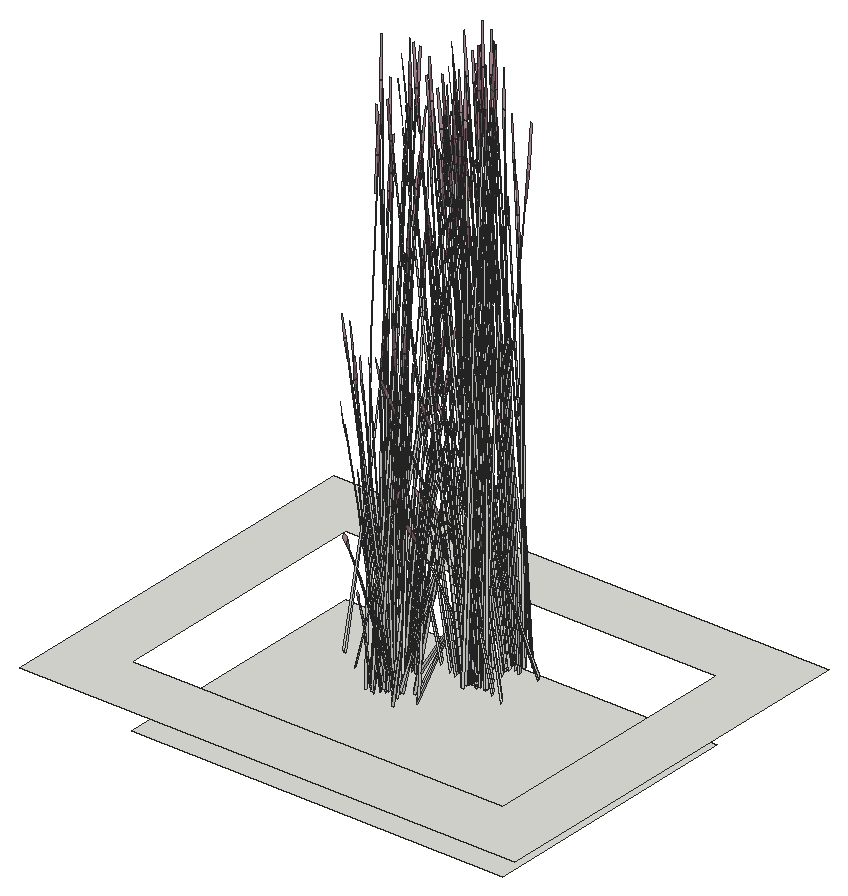
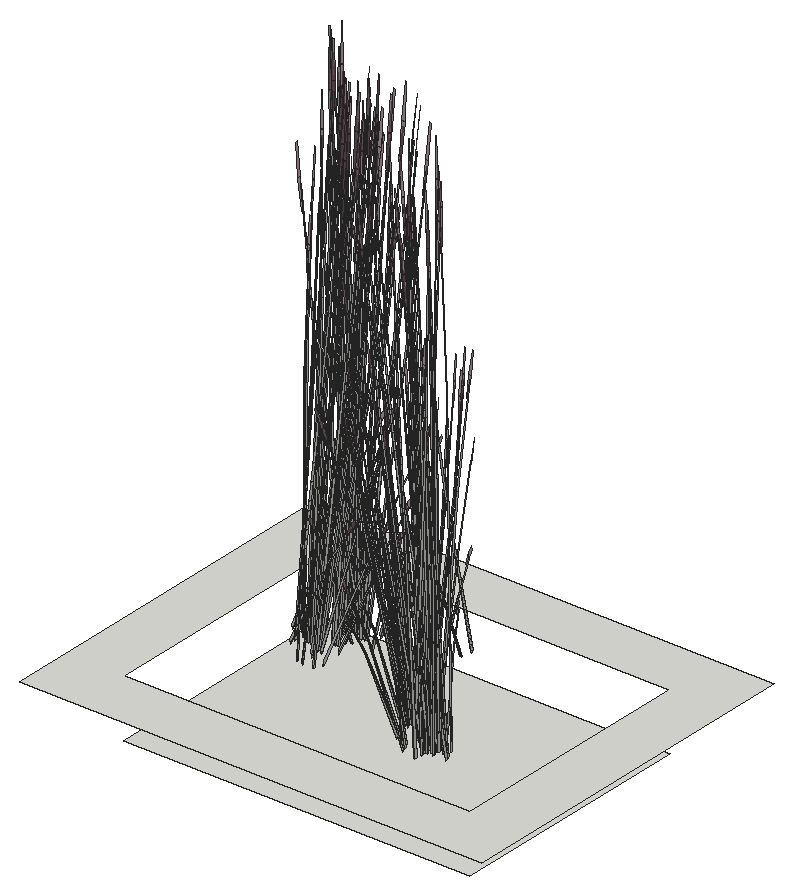
# SketchUp Ruby script. Lengths in inches.
U = 1.inch
M = Sketchup.active_model
def pt(a) = Geom::Point3d.new(a.map { |v| v * U })
def face(e, loops, mat)
  f = e.add_face(loops[0].map { |a| pt(a) })
  loops[1..].each { |l| e.add_face(l.map { |a| pt(a) }).erase! }
  f.material = f.back_material = mat if mat
  f
end
# faces: each face lists its corners as indices into pts; further lists are holes
def faces(e, pts, list, mat = nil) = list.each { |f| face(e, (f[0].is_a?(Array) ? f : [f]).map { |l| l.map { |i| pts[i] } }, mat) }
# xy, xz, yz: faces in a plane at the given z, y or x. An outline is a flat list of corners, or four numbers for a rectangle; further outlines are holes
def ring(l) = l.size == 4 ? [[l[0], l[1]], [l[2], l[1]], [l[2], l[3]], [l[0], l[3]]] : l.each_slice(2).to_a
def flat(e, list, mat, &to3) = list.each { |f| face(e, (f[0].is_a?(Array) ? f : [f]).map { |l| ring(l).map { |u, v| to3.(u, v) } }, mat) }
def xy(e, z, list, mat = nil) = flat(e, list, mat) { |x, y| [x, y, z] }
def xz(e, y, list, mat = nil) = flat(e, list, mat) { |x, z| [x, y, z] }
def yz(e, x, list, mat = nil) = flat(e, list, mat) { |y, z| [x, y, z] }
def lines(e, pts, list) = list.each { |a, b| e.add_line(pt(pts[a]), pt(pts[b])) }
# prism: a flat outline (further loops are holes) pulled along v
def prism(e, loops, v, mat = nil)
  f = face(e, loops, mat); d = Geom::Vector3d.new(v.map { |x| x * U })
  f.pushpull(f.normal.samedirection?(d) ? d.length : -d.length)
end
def box(e, o, s, mat = nil) = prism(e, [[o, [o[0] + s[0], o[1], o[2]], [o[0] + s[0], o[1] + s[1], o[2]], [o[0], o[1] + s[1], o[2]]]], [0, 0, s[2]], mat)
def at(x, y, z, deg = 0) = Geom::Transformation.translation(pt([x, y, z])) * Geom::Transformation.rotation(ORIGIN, Z_AXIS, deg.degrees)
def axes(o, x, y, z) = Geom::Transformation.new([*x, 0, *y, 0, *z, 0, *pt(o).to_a, 1])
def part(name) = M.definitions.add(name)
# library, detail: a bought-in or finely detailed component or shape, given as its bounding box
def library(name, o, s) = part(name).tap { |d| box(d.entities, o, s) }
def detail(e, o, s) = box(e.add_group.entities, o, s)
def put(e, d, t, mat = nil) = e.add_instance(d, t).tap { |i| i.material = mat if mat }
def group(e, t, mat = nil) = e.add_group.tap { |g| g.transformation = t; g.material = mat if mat }.entities
root = M.entities
M.materials.add("LightPink_Translucent").color = [144, 107, 117]
M.materials["LightPink_Translucent"].alpha = 0.75
c1 = part("blade")
p = [[2.15,0.21,22],[0,0.17,0],[0.09,0.45,0],[2.18,0.31,22],[2.29,0.31,22],[0.38,0.45,0],
  [2.48,0.24,33],[2.49,0.24,33],[2.48,0.22,33]]
faces(c1.entities,p,[[0,1,2,3],[4,5,2,3],[6,3,4,7],[8,0,3,6]])
c2 = part("seeds")
p = [[0.3,-0.1,1.38],[-0.01,-0.03,1.59],[-0.01,-0.03,0.03],[0.14,-0.07,-0.07],[0.29,-0.03,3],[0.15,0.01,3.11]]
faces(c2.entities,p,[[0,1,2,3],[1,0,4,5]],"LightPink_Translucent")
c3 = part("blade with seeds")
put(c3.entities,c1,at(0,0,0))
put(c3.entities,c2,axes([2.4,0.25,30.99],[1.5799,-0.05474,1.17369],[-0.12525,1.92788,0.29478],[-0.07173,-0.02425,1.56792]))
xy(root,42,[[310,14,346,40]])
xy(root,48,[[[304,8,352,46],[310,14,346,40]]])
put(root,c3,axes([323.19,27.42,46.18],[0.37205,-0.1328,0.05682],[0.18211,0.24217,0.44729],[-0.03593,-0.10675,0.68204]))
put(root,c3,axes([324.42,29.2,44.1875],[-0.39671,-0.28463,0.15589],[0.39978,-0.27607,0.31002],[-0.04381,0.05813,1.41735]))
put(root,c3,axes([323.05,29.04,43.95],[0,-0.45213,0],[0.63136,0,0],[0,0,1.58567]))
put(root,c3,axes([323.0625,27.45,46.18],[0.49753,0.10215,0.42415],[-0.17013,0.33585,0.34973],[-0.0299,-0.13207,0.87768]))
put(root,c3,axes([322.47,29.12,44.15],[0.56891,0.18939,0.21263],[-0.2738,0.39352,0.44182],[0,-0.09071,1.41855]))
put(root,c3,axes([322.28,28.86,44.4],[-0.54829,0.02412,0.39531],[-0.04958,-0.40041,-0.19025],[0.09816,-0.04058,1.26923]))
put(root,c3,axes([322.03,28.17,44.1875],[-0.14586,0.38834,0.15589],[-0.53375,-0.1099,0.31002],[0.0922,-0.00189,1.41735]))
put(root,c3,axes([321.77,27.69,44.1],[-0.31568,-0.39156,0],[0.52815,-0.21836,-0.456],[0.12029,-0.04973,1.44655]))
put(root,c3,axes([323.64,28.19,44.1875],[-0.54257,0.10371,0.15589],[-0.13397,-0.38597,0.31002],[0.04839,0.05624,1.41735]))
put(root,c3,axes([323.09,26.74,44.44],[0.06477,0.22786,1.01491],[-0.35932,-0.1262,0.74569],[0.03867,-0.11667,0.22354]))
put(root,c3,axes([322.75,28.75,44.09],[-0.41865,0.35461,0.40429],[-0.49737,-0.31303,0.15865],[0.10093,-0.03539,1.40366]))
put(root,c3,axes([323.47,29.3125,43.96],[0.35245,0.2524,0],[-0.35245,0.2524,0],[0,0,1.49564]))
put(root,c3,axes([323.3,28.93,44.1],[-0.63817,-0.08233,0.43472],[0.12987,-0.46497,0.17059],[0.09326,0.0449,1.50931]))
put(root,c3,axes([323.94,22.14,50.49],[0.45869,-0.0692,0.0575],[0.10545,0.27878,-0.76259],[-0.02908,0.14112,0.68355]))
put(root,c3,axes([324.625,27.12,46.16],[-0.05128,0.02985,1.56736],[-0.5024,-0.1007,-0.1481],[-0.01819,-0.13025,0.27737]))
put(root,c3,axes([324.23,27.98,46.45],[-0.55492,-0.01936,-0.10745],[0.01517,-0.36657,-0.59638],[0.03855,-0.14118,0.90619]))
put(root,c3,axes([323.48,29.14,43.95],[0.56491,0,0],[0,0.40454,0],[0,0,1.5764]))
put(root,c3,axes([324.01,28.03,46.46],[-0.34164,0.20573,0.31292],[-0.3234,-0.23491,-0.40398],[0.04921,-0.11936,0.77298]))
put(root,c3,axes([322.9375,28.69,44.4],[-0.30332,-0.32798,0.39531],[0.45944,-0.23096,-0.19025],[0.09816,0.04058,1.26923]))
put(root,c3,axes([322.39,28.77,44.36],[-0.05884,-0.44587,-0.25709],[0.6128,-0.02696,-0.44182],[0.10791,-0.05939,1.41118]))
put(root,c3,axes([323.85,27.84,46.14],[-0.36145,-0.26255,-0.45151],[0.38183,-0.22994,-0.34973],[0.055,-0.1334,0.86392]))
put(root,c3,axes([322.31,27.78,43.79],[0.47106,0.09668,-0.27372],[-0.11861,0.34048,0.27372],[0.09497,-0.03926,1.22797]))
put(root,c3,axes([323.62,27.375,44.29],[-0.14352,0.07909,1.26356],[-0.42983,-0.13843,-0.27174],[0.07968,-0.17216,0.54024]))
put(root,c3,axes([322.19,27.63,43.78],[0.47255,-0.19538,-0.43871],[0.28245,0.35034,0],[0.10763,-0.0445,1.3917]))
put(root,c3,axes([323.14,28.6,44.3125],[0.09741,-0.34873,0.12794],[0.4759,0.06053,-0.36534],[0.08661,0.03581,1.11991]))
put(root,c3,axes([323.82,27.99,44.19],[-0.47255,-0.19538,0.43871],[0.28245,-0.35034,0],[0.10763,0.0445,1.3917]))
put(root,c3,axes([323.97,27.96,46.4],[0.01314,-0.36145,-0.62776],[0.55324,0.02428,0.07576],[0.05838,-0.15313,0.88802]))
put(root,c3,axes([323.41,30.03,43.93],[0.53009,-0.13258,-0.16963],[0.18627,0.38191,0.00007],[0.05851,-0.01465,1.53656]))
put(root,c3,axes([325.07,22.08,49.32],[0.08172,-0.02126,1.55816],[0.49154,0.11703,-0.23804],[0.01437,0.1319,0.26541]))
put(root,c3,axes([324.19,27.74,46],[0.34164,-0.20573,-0.31292],[0.3234,0.23491,0.40398],[0.04921,-0.11936,0.77298]))
put(root,c3,axes([324.32,27.85,46.18],[0.41493,0.01821,0.05682],[-0.01138,0.27493,0.44729],[0.04342,-0.10531,0.68204]))
put(root,c3,axes([324.74,27.39,46.17],[-0.00487,-0.07777,1.54581],[-0.41166,-0.22476,-0.24447],[0.06364,-0.13625,0.12397]))
put(root,c3,axes([322.76,28.43,43.82],[0.34009,-0.2937,-0.55095],[0.42248,0.26632,-0.1446],[0.13628,-0.07327,1.21613]))
put(root,c3,axes([324.19,27.82,46.18],[0.35954,0.26661,0.42415],[-0.38183,0.22994,0.34973],[0.06632,-0.12508,0.87768]))
put(root,c3,axes([324.25,28.17,43.79],[0.11861,0.34048,-0.27372],[-0.47106,0.09668,0.27372],[0.09497,0.03926,1.22797]))
put(root,c3,axes([323.09,28.71,44.36],[0.50979,-0.25942,-0.25709],[0.339,0.36656,-0.44182],[0.12578,0.03723,1.41118]))
put(root,c3,axes([324.61,28.67,46.46],[-0.43951,0.05584,0.31292],[-0.11606,-0.31924,-0.40398],[0.12595,-0.08575,0.77298]))
put(root,c3,axes([323.34,27.78,45.43],[-0.09401,0.13431,1.51428],[-0.3944,-0.27795,0.12244],[0.17792,-0.17323,0.64734]))
put(root,c3,axes([321.81,28.48,43.41],[-0.49699,0.15644,1.13921],[-0.15819,-0.44887,0.44265],[0.30518,0.00747,1.29573]))
put(root,c3,axes([324.84,28.7,46.45],[-0.46706,-0.21546,-0.10745],[0.26908,-0.31203,-0.59638],[0.13196,-0.10846,0.90619]))
put(root,c3,axes([324.09,27.79,44.1],[0.31568,-0.39156,0],[0.52815,0.21836,-0.456],[0.12029,0.04973,1.44655]))
put(root,c3,axes([324.62,27.62,43.32],[-0.07557,-0.03078,1.55816],[-0.19412,-0.34391,-0.23804],[0.13095,-0.09333,0.26541]))
put(root,c3,axes([324.38,28.02,43.78],[0.47255,0.19538,-0.43871],[-0.28245,0.35034,0],[0.10763,0.0445,1.3917]))
put(root,c3,axes([331.07,25.07,50.29],[0.17547,0.03208,1.26356],[0.1131,0.32764,-0.27174],[-0.23835,0.06133,0.54024]))
put(root,c3,axes([324.6,28.44,46.14],[-0.12971,-0.3568,-0.45151],[0.49122,-0.06241,-0.34973],[0.14077,-0.09583,0.86392]))
put(root,c3,axes([324.68,29.43,46.46],[-0.41962,-0.10901,0.31292],[0.12239,-0.31802,-0.40398],[0.16894,-0.02916,0.77298]))
put(root,c3,axes([323.6875,28.77,43.82],[0.52523,0.06406,-0.55095],[-0.11084,0.39517,-0.1446],[0.15674,0.04788,1.21613]))
put(root,c3,axes([325.93,29.01,44],[-0.31304,-0.24986,-0.05733],[0.34284,-0.22894,-0.25992],[0.09714,-0.01612,0.85731]))
put(root,c3,axes([325.21,27.73,44.44],[-0.16818,0.19891,1.01491],[-0.14456,-0.26725,0.74569],[0.1389,-0.06697,0.22354]))
put(root,c3,axes([325.01,28.62,46.18],[0.34663,0.16434,0.05682],[-0.20181,0.23402,0.44729],[0.11113,-0.07566,0.68204]))
put(root,c3,axes([324.91,28.55,46.18],[0.12522,0.35963,0.42415],[-0.49122,0.06241,0.34973],[0.14477,-0.08458,0.87768]))
put(root,c3,axes([325.99,28.61,46.16],[-0.06595,-0.00297,1.56736],[-0.27386,-0.31799,-0.1481],[0.10998,-0.10455,0.27737]))
put(root,c3,axes([329.65,22.125,50.29],[0.15933,-0.06164,1.26356],[0.39339,0.18587,-0.27174],[-0.11709,0.16083,0.54024]))
put(root,c3,axes([324.97,28.48,46],[0.43951,-0.05584,-0.31292],[0.11606,0.31924,0.40398],[0.12595,-0.08575,0.77298]))
put(root,c3,axes([324.62,28.59,46.4],[0.26374,-0.30832,-0.62776],[0.46217,0.21911,0.07576],[0.15748,-0.11171,0.88802]))
put(root,c3,axes([325.06,29.53,46.18],[0.18545,0.26643,0.05682],[-0.33817,0.13041,0.44729],[0.14907,-0.02573,0.68204]))
put(root,c3,axes([324.85,29.54,46.45],[-0.25405,-0.35383,-0.10745],[0.45089,-0.17388,-0.59638],[0.19001,-0.04668,0.90619]))
put(root,c3,axes([325.02,29.4375,46.18],[-0.14265,0.35629,0.42415],[-0.46898,-0.12183,0.34973],[0.18443,-0.02141,0.87768]))
put(root,c3,axes([324.83,29.24,46.14],[0.13679,-0.35544,-0.45151],[0.46898,0.12183,-0.34973],[0.18882,-0.03259,0.86392]))
put(root,c3,axes([326.01,29.46,44.44],[-0.31197,0.06451,1.01491],[0.14684,-0.26661,0.74569],[0.1655,0.01824,0.22354]))
put(root,c3,axes([331.25,25.9375,49.32],[0.06773,0.03904,1.55816],[0.11484,0.36171,-0.23804],[-0.15011,0.07713,0.26541]))
put(root,c3,axes([325,28.3,44.29],[-0.18038,-0.01157,1.26356],[-0.18479,-0.31048,-0.27174],[0.22159,-0.08783,0.54024]))
put(root,c3,axes([325.12,29.4,46],[0.41962,0.10901,-0.31292],[-0.12239,0.31802,0.40398],[0.16894,-0.02916,0.77298]))
put(root,c3,axes([325.33,29.34,43.75],[-0.3252,0.04689,1.25103],[-0.05176,-0.37326,0.07161],[0.22777,-0.0565,0.71188]))
put(root,c3,axes([325.6875,29.09,43.32],[-0.02639,-0.05932,1.55816],[0.18302,-0.34702,-0.23804],[0.18462,-0.00499,0.26541]))
put(root,c3,axes([323.98,29,45.43],[-0.20943,0.00885,1.51428],[0.13893,-0.38357,0.12244],[0.29846,0.02372,0.64734]))
put(root,c3,axes([324.74,29.37,46.4],[0.44368,-0.17257,-0.62776],[0.24726,0.35524,0.07576],[0.21437,-0.04035,0.88802]))
put(root,c3,axes([333.59,27.25,50.29],[0.09858,0.10879,1.26356],[-0.22716,0.29571,-0.27174],[-0.23325,-0.07068,0.54024]))
put(root,c3,axes([326.23,28.99,46.17],[0.07006,-0.05952,1.54581],[-0.08968,-0.3651,-0.24447],[0.1758,-0.06922,0.12397]))
put(root,c3,axes([332.39,25.52,49.78],[-0.47255,-0.19538,-0.43871],[0.28245,-0.35034,0],[-0.10763,-0.0445,1.3917]))
put(root,c3,axes([333.24,27.98,49.32],[0.0128,0.06158,1.55816],[-0.25814,0.3216,-0.23804],[-0.18336,-0.01621,0.26541]))
put(root,c3,axes([332.68,25.75,50.1],[-0.31568,0.39156,0],[-0.52815,-0.21836,-0.456],[-0.12029,-0.04973,1.44655]))
put(root,c3,axes([332.1,26.32,50.29],[0.15933,-0.06164,1.26356],[0.39339,0.18587,-0.27174],[-0.11709,0.16083,0.54024]))
put(root,c3,axes([333.68,24.83,50.36],[-0.50979,0.25942,-0.25709],[-0.339,-0.36656,-0.44182],[-0.12578,-0.03723,1.41118]))
put(root,c3,axes([333.12,30.35,49.32],[-0.04891,0.05148,1.55816],[-0.49427,0.11098,-0.23804],[-0.1194,-0.10096,0.26541]))
put(root,c3,axes([334.02,25.11,49.82],[-0.34009,0.2937,-0.55095],[-0.42248,-0.26632,-0.1446],[-0.13628,0.07327,1.21613]))
put(root,c3,axes([334.25,24.95,50.18],[-0.49304,-0.31451,-0.2226],[0.41487,-0.35316,0.48713],[-0.13277,0.03679,1.48635]))
put(root,c3,axes([334.92,28.54,49.82],[-0.52523,-0.06406,-0.55095],[0.11084,-0.39517,-0.1446],[-0.15674,-0.04788,1.21613]))
put(root,c3,axes([334,24.88,49.95],[-0.54829,0.02412,-0.39531],[-0.04958,-0.40041,0.19025],[-0.09816,0.04058,1.26923]))
put(root,c3,axes([333.48,30.15,50.29],[-0.03058,0.12783,1.26356],[-0.44698,0.10701,-0.27174],[-0.10448,-0.16522,0.54024]))
put(root,c3,axes([332.95,25.55,50.19],[0.47255,0.19538,0.43871],[-0.28245,0.35034,0],[-0.10763,-0.0445,1.3917]))
put(root,c3,axes([334.24,29.29,49.78],[-0.47255,-0.19538,-0.43871],[0.28245,-0.35034,0],[-0.10763,-0.0445,1.3917]))
put(root,c3,axes([334.03,26.38,49.32],[-0.04891,0.05148,1.55816],[-0.49427,0.11098,-0.23804],[-0.1194,-0.10096,0.26541]))
put(root,c3,axes([334.52,29.53,50.1],[-0.31568,0.39156,0],[-0.52815,-0.21836,-0.456],[-0.12029,-0.04973,1.44655]))
put(root,c3,axes([333.63,24.94,50.3125],[-0.09741,0.34873,0.12794],[-0.4759,-0.06053,-0.36534],[-0.08661,-0.03581,1.11991]))
put(root,c3,axes([334.58,25.91,49.78],[-0.47255,0.19538,-0.43871],[-0.28245,-0.35034,0],[-0.10763,0.0445,1.3917]))
put(root,c3,axes([334.61,25.81,49.9375],[-0.31175,-0.39292,-0.04544],[0.52815,-0.21836,0.456],[-0.13015,0.03741,1.44584]))
put(root,c3,axes([334.46,25.76,49.79],[-0.47106,-0.09668,-0.27372],[0.11861,-0.34048,0.27372],[-0.09497,0.03926,1.22797]))
put(root,c3,axes([333.72,26.58,49.88],[-0.14565,0.31907,-0.0344],[-0.44829,-0.09815,-0.15595],[-0.06806,-0.05219,0.51438]))
put(root,c3,axes([332.21,26.02,50.49],[0.45869,-0.0692,0.0575],[0.10545,0.27878,-0.76259],[-0.02908,0.14112,0.68355]))
put(root,c3,axes([334.38,24.77,50.36],[0.05884,0.44587,-0.25709],[-0.6128,0.02696,-0.44182],[-0.10791,0.05939,1.41118]))
put(root,c3,axes([335.52,28.6,50.36],[-0.50979,0.25942,-0.25709],[-0.339,-0.36656,-0.44182],[-0.12578,-0.03723,1.41118]))
put(root,c3,axes([333.48,28.03,50.1],[-0.63136,0,0],[0,-0.43672,-0.456],[0,-0.09947,1.44655]))
put(root,c3,axes([334.37,29.14,49.79],[-0.11861,-0.34048,-0.27372],[0.47106,-0.09668,0.27372],[-0.09497,-0.03926,1.22797]))
put(root,c3,axes([332.71,31.71,49.78],[0,-0.39075,-0.43871],[0.56491,0,0],[0,-0.089,1.3917]))
put(root,c3,axes([333.97,27.92,50.06],[-0.46965,0.32852,0.27176],[-0.46994,-0.32506,-0.32244],[-0.0164,-0.09329,1.45692]))
put(root,c3,axes([337.07,23.74,50.29],[0.17547,0.03208,1.26356],[0.1131,0.32764,-0.27174],[-0.23835,0.06133,0.54024]))
put(root,c3,axes([336.09,28.72,50.18],[-0.49304,-0.31451,-0.2226],[0.41487,-0.35316,0.48713],[-0.13277,0.03679,1.48635]))
put(root,c3,axes([335.2,28.42,49.95],[-0.30332,-0.32798,-0.39531],[0.45944,-0.23096,0.19025],[-0.09816,-0.04058,1.26923]))
put(root,c3,axes([333.83,25.41,49.94],[-0.50902,-0.17543,0],[0.24498,-0.36452,0],[0,0,1.43768]))
put(root,c3,axes([335,25.85,50.1],[0.31568,0.39156,0],[-0.52815,0.21836,-0.456],[-0.12029,0.04973,1.44655]))
put(root,c3,axes([335.84,28.65,49.95],[-0.54829,0.02412,-0.39531],[-0.04958,-0.40041,0.19025],[-0.09816,0.04058,1.26923]))
put(root,c3,axes([333.93,31.77,49.85],[-0.20736,-0.4007,-0.61707],[0.59731,-0.14431,-0.16195],[-0.02292,-0.13569,1.36206]))
put(root,c3,axes([334.74,25.37,50.1875],[0.14586,-0.38834,0.15589],[0.53375,0.1099,0.31002],[-0.0922,0.00189,1.41735]))
put(root,c3,axes([334.5,24.86,50.3125],[0.37303,0.23477,0.12794],[-0.31115,0.26487,-0.36534],[-0.08661,0.03581,1.11991]))
put(root,c3,axes([334.8,29.32,50.19],[0.47255,0.19538,0.43871],[-0.28245,0.35034,0],[-0.10763,-0.0445,1.3917]))
put(root,c3,axes([334.49,24.69,50.4],[0.54829,-0.02412,0.39531],[0.04958,0.40041,-0.19025],[-0.09816,0.04058,1.26923]))
put(root,c3,axes([335.24,28.6,50.16],[0.13383,-0.46302,-0.20702],[0.63453,0.08071,0.45303],[-0.11087,-0.06394,1.38231]))
put(root,c3,axes([334.55,30.14,49.88],[-0.34892,0.22417,-0.0344],[-0.3197,-0.24551,-0.15595],[-0.02251,-0.06957,0.51438]))
put(root,c3,axes([334.62,25.61,50.06],[0.63212,0.12701,0.27176],[-0.15814,0.45398,-0.32244],[-0.10462,0.05682,1.45692]))
put(root,c3,axes([337.74,28.35,50.29],[0.09858,0.10879,1.26356],[-0.22716,0.29571,-0.27174],[-0.23325,-0.07068,0.54024]))
put(root,c3,axes([335.47,28.71,50.3125],[-0.09741,0.34873,0.12794],[-0.4759,-0.06053,-0.36534],[-0.08661,-0.03581,1.11991]))
put(root,c3,axes([334.89,25.58,50.19],[0.47255,-0.19538,0.43871],[0.28245,0.35034,0],[-0.10763,0.0445,1.3917]))
put(root,c3,axes([333.62,27.74,49.78],[0,-0.39075,-0.43871],[0.56491,0,0],[0,-0.089,1.3917]))
put(root,c3,axes([333.86,28.1,50.19],[0,0.39075,0.43871],[-0.56491,0,0],[0,-0.089,1.3917]))
put(root,c3,axes([336.45,29.58,49.9375],[-0.31175,-0.39292,-0.04544],[0.52815,-0.21836,0.456],[-0.13015,0.03741,1.44584]))
put(root,c3,axes([333.94,25.26,49.95],[-0.16474,-0.33688,0],[0.47043,-0.11798,0],[0,0,1.36402]))
put(root,c3,axes([333.34,25.97,49.32],[0.08172,-0.02126,1.55816],[0.49154,0.11703,-0.23804],[0.01437,0.1319,0.26541]))
put(root,c3,axes([335.1,28.19,50.36],[-0.56863,-0.18645,-0.25709],[0.2738,-0.39352,-0.44182],[-0.01787,-0.09662,1.41118]))
put(root,c3,axes([337.39,29.08,49.32],[0.0128,0.06158,1.55816],[-0.25814,0.3216,-0.23804],[-0.18336,-0.01621,0.26541]))
put(root,c3,axes([334.61,24.6,49.95],[-0.24498,0.3521,-0.39531],[-0.50902,-0.16945,0.19025],[0,0.08116,1.26923]))
put(root,c3,axes([334.84,27.79,49.85],[-0.20736,-0.4007,-0.61707],[0.59731,-0.14431,-0.16195],[-0.02292,-0.13569,1.36206]))
put(root,c3,axes([335.58,24.38,50.1875],[-0.39671,-0.28463,0.15589],[0.39978,-0.27607,0.31002],[-0.04381,0.05813,1.41735]))
put(root,c3,axes([334.52,24.4,50.03],[0,0.45191,-0.04981],[-0.63136,0,0],[0,0.0142,1.58489]))
put(root,c3,axes([333.86,27.75,49.79],[0.35245,-0.2438,-0.27372],[0.35245,0.2438,0.27372],[0,-0.07853,1.22797]))
put(root,c3,axes([335.46,26.17,49.88],[-0.34892,0.22417,-0.0344],[-0.3197,-0.24551,-0.15595],[-0.02251,-0.06957,0.51438]))
put(root,c3,axes([335.31,28.38,50.09],[0.63817,0.08233,0.40429],[-0.12987,0.46497,0.15865],[-0.09326,-0.0449,1.40366]))
put(root,c3,axes([334.22,25.27,50.02],[0.21952,0.44891,-0.05313],[-0.62724,0.1573,0],[0.00767,0.01568,1.52132]))
put(root,c3,axes([334.63,29.87,49.32],[-0.08469,0.01408,1.55816],[-0.46834,-0.15847,-0.23804],[0.00786,-0.13218,0.26541]))
put(root,c3,axes([337.25,24.61,49.32],[0.06773,0.03904,1.55816],[0.11484,0.36171,-0.23804],[-0.15011,0.07713,0.26541]))
put(root,c3,axes([335.15,28.3,50.4],[-0.24498,0.3521,0.39531],[-0.50902,-0.16945,-0.19025],[0,-0.08116,1.26923]))
put(root,c3,axes([334.25,31.87,49.95],[0.24498,-0.3521,-0.39531],[0.50902,0.16945,0.19025],[0,-0.08116,1.26923]))
put(root,c3,axes([336.03,24.68,49.94],[-0.63105,-0.00312,-0.04397],[0,-0.43672,0.44129],[-0.01983,0.09942,1.3992]))
put(root,c3,axes([334.79,23.37,50.1875],[-0.54257,0.10371,0.15589],[-0.13397,-0.38597,0.31002],[0.04839,0.05624,1.41735]))
put(root,c3,axes([334.97,29.125,50.1875],[0.54257,-0.10371,0.15589],[0.13397,0.38597,0.31002],[-0.04839,-0.05624,1.41735]))
put(root,c3,axes([335.67,29.19,49.94],[-0.50902,-0.17543,0],[0.24498,-0.36452,0],[0,0,1.43768]))
put(root,c3,axes([334.62,24.49,49.96],[0.35245,0.2524,0],[-0.35245,0.2524,0],[0,0,1.49564]))
put(root,c3,axes([334.62,24.2,50.4],[0.24498,-0.3521,0.39531],[0.50902,0.16945,-0.19025],[0,0.08116,1.26923]))
put(root,c3,axes([334.4,25.42,49.95],[0.50902,0.17543,0],[-0.24498,0.36452,0],[0,0,1.54589]))
put(root,c3,axes([336.59,29.14,50.1875],[0.14586,-0.38834,0.15589],[0.53375,0.1099,0.31002],[-0.0922,0.00189,1.41735]))
put(root,c3,axes([336.34,28.63,50.3125],[0.37303,0.23477,0.12794],[-0.31115,0.26487,-0.36534],[-0.08661,0.03581,1.11991]))
put(root,c3,axes([334.45,24.11,50.1],[-0.63817,-0.08233,0.43472],[0.12987,-0.46497,0.17059],[0.09326,0.0449,1.50931]))
put(root,c3,axes([335.9,24.75,49.79],[-0.35245,0.2438,-0.27372],[-0.35245,-0.2438,0.27372],[0,0.07853,1.22797]))
put(root,c3,axes([336.21,28.34,50.03],[-0.46965,-0.33633,-0.05417],[0.46994,-0.33653,0],[-0.0164,-0.01174,1.55135]))
put(root,c3,axes([336.33,28.46,50.4],[0.54829,-0.02412,0.39531],[0.04958,0.40041,-0.19025],[-0.09816,0.04058,1.26923]))
put(root,c3,axes([334.9,24.7,49.85],[0.18514,0.35777,-0.61156],[-0.53331,0.12885,-0.16051],[0.02046,0.12115,1.3499]))
